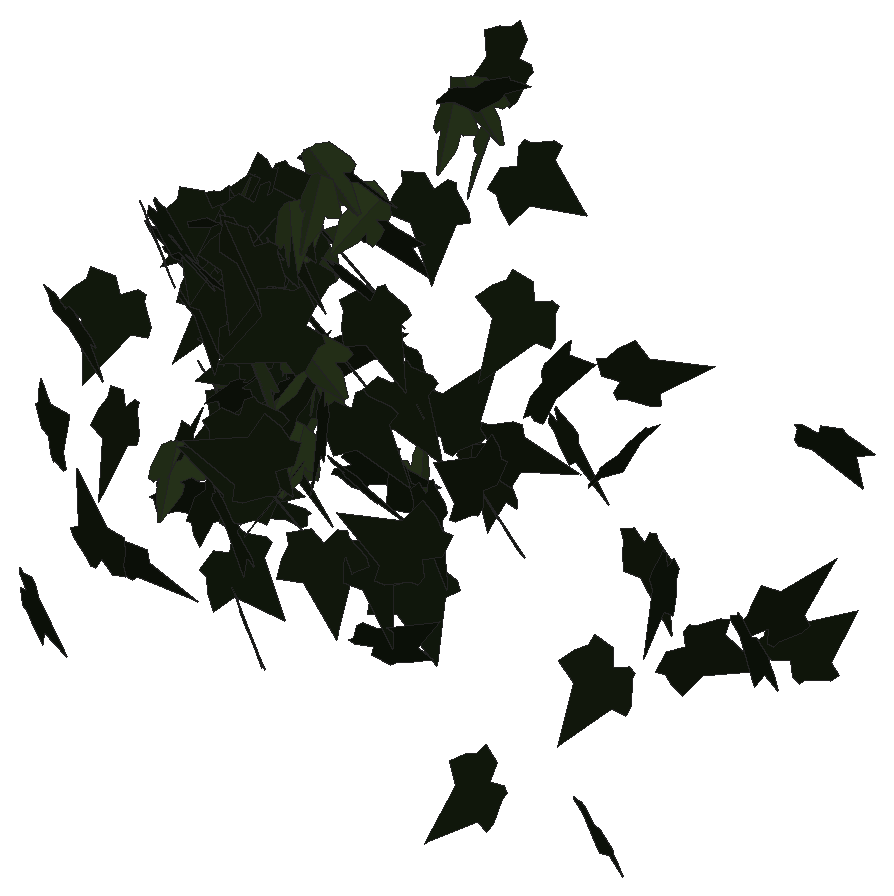
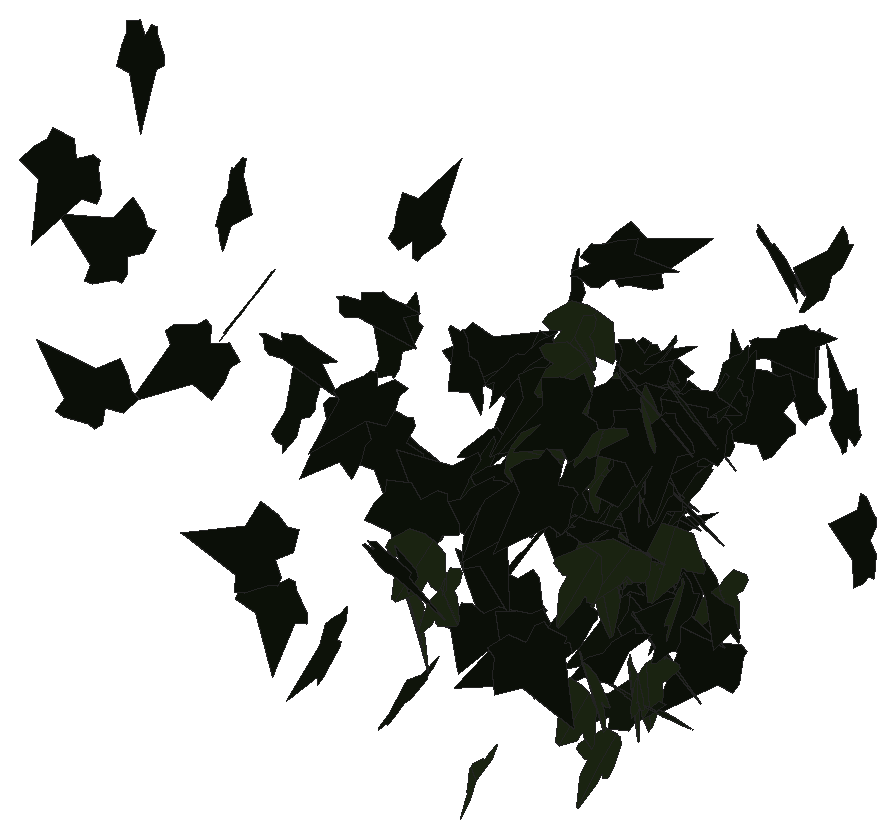
# SketchUp Ruby script. Lengths in inches.
U = 1.inch
M = Sketchup.active_model
def pt(a) = Geom::Point3d.new(a.map { |v| v * U })
def face(e, loops, mat)
  f = e.add_face(loops[0].map { |a| pt(a) })
  loops[1..].each { |l| e.add_face(l.map { |a| pt(a) }).erase! }
  f.material = f.back_material = mat if mat
  f
end
# faces: each face lists its corners as indices into pts; further lists are holes
def faces(e, pts, list, mat = nil) = list.each { |f| face(e, (f[0].is_a?(Array) ? f : [f]).map { |l| l.map { |i| pts[i] } }, mat) }
# xy, xz, yz: faces in a plane at the given z, y or x. An outline is a flat list of corners, or four numbers for a rectangle; further outlines are holes
def ring(l) = l.size == 4 ? [[l[0], l[1]], [l[2], l[1]], [l[2], l[3]], [l[0], l[3]]] : l.each_slice(2).to_a
def flat(e, list, mat, &to3) = list.each { |f| face(e, (f[0].is_a?(Array) ? f : [f]).map { |l| ring(l).map { |u, v| to3.(u, v) } }, mat) }
def xy(e, z, list, mat = nil) = flat(e, list, mat) { |x, y| [x, y, z] }
def xz(e, y, list, mat = nil) = flat(e, list, mat) { |x, z| [x, y, z] }
def yz(e, x, list, mat = nil) = flat(e, list, mat) { |y, z| [x, y, z] }
def lines(e, pts, list) = list.each { |a, b| e.add_line(pt(pts[a]), pt(pts[b])) }
# prism: a flat outline (further loops are holes) pulled along v
def prism(e, loops, v, mat = nil)
  f = face(e, loops, mat); d = Geom::Vector3d.new(v.map { |x| x * U })
  f.pushpull(f.normal.samedirection?(d) ? d.length : -d.length)
end
def box(e, o, s, mat = nil) = prism(e, [[o, [o[0] + s[0], o[1], o[2]], [o[0] + s[0], o[1] + s[1], o[2]], [o[0], o[1] + s[1], o[2]]]], [0, 0, s[2]], mat)
def at(x, y, z, deg = 0) = Geom::Transformation.translation(pt([x, y, z])) * Geom::Transformation.rotation(ORIGIN, Z_AXIS, deg.degrees)
def axes(o, x, y, z) = Geom::Transformation.new([*x, 0, *y, 0, *z, 0, *pt(o).to_a, 1])
def part(name) = M.definitions.add(name)
# library, detail: a bought-in or finely detailed component or shape, given as its bounding box
def library(name, o, s) = part(name).tap { |d| box(d.entities, o, s) }
def detail(e, o, s) = box(e.add_group.entities, o, s)
def put(e, d, t, mat = nil) = e.add_instance(d, t).tap { |i| i.material = mat if mat }
def group(e, t, mat = nil) = e.add_group.tap { |g| g.transformation = t; g.material = mat if mat }.entities
root = M.entities
M.materials.add("efeu1").color = [18, 25, 13]
M.materials.add("efeu2").color = [43, 57, 29]
c1 = part("ivyleaf_10")
p = [[0,0.5,-0.03],[-0.0625,2.02,-0.43],[-0.19,2.01,-0.46],[-0.54,1.05,-0.29],[-0.52,0.625,-0.18],[-0.83,0.76,-0.28],
  [-1.16,0.64,-0.33],[-1.15,0.33,-0.24],[-0.77,-0.39,0.02],[-0.3,-0.51,0.16],[0.04,-0.48,0.23],[-0.02,2.01,-0.4375],
  [-0.06,2.01,-0.43],[0.04,-0.49,0.23],[0.67,-0.49,0.14],[1.38,0.36,-0.2],[1.375,0.51,-0.24],[0.81,0.65,-0.19],
  [0.62,0.59,-0.15],[0.6,1.09,-0.28],[0.5,1.23,-0.31]]
faces(c1.entities,p,[[0,1,2,3,4,5,6,7,8,9,10],[11,12,0,13,14,15,16,17,18,19,20]],"efeu2")
c2 = part("ivyleaf_9")
p = [[1.54,2.16,1.25],[1.36,2.04,1.19],[-0.21,0.99,0.68],[-0.71,1.11,0.82],[-0.85,0.86,0.67],[-0.8,0.17,0.21],
  [-0.9,-0.01,0.1],[-0.67,-0.16,-0.02],[-0.08,-0.08,-0.05],[-0.03,-0.6,-0.4],[0.65,-0.88,-0.66],[0.83,-0.6,-0.49],
  [1.29,-0.42,-0.43],[1.8125,-0.07,-0.26],[1.21,0.44,0.15]]
faces(c2.entities,p,[[0,1,2,3,4,5,6,7,8,9,10,11,12,13,14]],"efeu1")
put(root,c1,axes([53.33,221.73,244.58],[-0.26084,0.4133,0.10556],[-0.07736,0.07585,-0.48812],[-0.4195,-0.27098,0.02438]))
put(root,c1,axes([53.07,223.4,246.125],[0.30993,0.29947,0.2535],[0.18973,0.16837,-0.43087],[-0.34343,0.36327,-0.00928]))
put(root,c1,axes([53.33,223.49,242.65],[-0.0186,0.35996,0.34653],[-0.09177,0.33841,-0.35645],[-0.49115,-0.07687,0.05348]))
put(root,c2,axes([53.1,220.57,248.04],[0.41377,-0.25598,-0.11519],[-0.07624,0.09498,-0.48494],[0.27015,0.41887,0.03957]))
put(root,c1,axes([53.34,221.92,245.64],[-0.47378,-0.13933,-0.07822],[0.06988,0.03944,-0.49352],[0.14369,-0.47857,-0.0179]))
put(root,c2,axes([53.54,220.39,243.92],[-0.03647,0.33293,0.37125],[-0.07657,0.36409,-0.33403],[-0.49276,-0.08121,0.02443]))
put(root,c2,axes([53.12,220.46,247.59],[-0.00979,-0.13779,0.48054],[0.15986,-0.45626,-0.12757],[0.47366,0.15114,0.05298]))
put(root,c2,axes([53.24,221.18,247.5625],[0.42087,0.26197,0.06512],[0.04723,0.04729,-0.49551],[-0.26578,0.42324,0.01506]))
put(root,c1,axes([53.41,223.85,245.99],[0.07815,0.31695,0.37873],[-0.09983,0.38566,-0.30215],[-0.48366,-0.02839,0.12357]))
put(root,c2,axes([53.68,221.22,247.84],[-0.43329,0.24928,0.01071],[-0.00923,0.00543,-0.49989],[-0.24934,-0.43339,-0.0001]))
put(root,c2,axes([53,220.875,247.33],[0.30392,-0.2346,0.32031],[0.28266,-0.15543,-0.38203],[0.27882,0.41329,0.03814]))
put(root,c2,axes([53.57,221.66,246.39],[-0.48347,0.01902,-0.12608],[0.12235,-0.06993,-0.47973],[-0.03588,-0.49472,0.06296]))
put(root,c2,axes([53.52,222.16,247.72],[0.18179,0.42237,-0.19635],[-0.07659,-0.1808,-0.45983],[-0.45944,0.19726,-0.00104]))
put(root,c2,axes([53.08,222.02,244.29],[0.27728,-0.31054,0.27692],[0.18201,-0.20872,-0.41631],[0.37415,0.33166,-0.0027]))
put(root,c1,axes([53.48,227.42,247.08],[0.00599,0.42329,-0.26606],[-0.03576,-0.26503,-0.42247],[-0.49868,0.02409,0.0271]))
put(root,c2,axes([53.61,222.16,246.78],[0.10913,0.48615,-0.04178],[-0.00362,-0.04201,-0.49822],[-0.48793,0.10904,-0.00565]))
put(root,c2,axes([53.49,221.3125,247.93],[-0.34329,-0.32192,-0.16886],[0.14758,0.08884,-0.46939],[0.33222,-0.37212,0.03402]))
put(root,c1,axes([53.48,222.25,243.3],[0.0044,-0.49057,0.09654],[0.15238,-0.09063,-0.46751],[0.47619,0.03353,0.14871]))
put(root,c1,axes([53.54,220.37,243.96],[0.09196,0.44535,-0.20786],[-0.0654,-0.1985,-0.45423],[-0.4871,0.11073,0.02174]))
put(root,c1,axes([53.55,223.64,243.95],[0.40572,-0.2915,-0.02053],[-0.01458,0.0149,-0.49957],[0.29186,0.40596,0.00359]))
put(root,c2,axes([53.42,220.58,243.18],[0.39535,0.29035,0.09693],[0.07144,0.06644,-0.49039],[-0.29765,0.4016,0.01105]))
put(root,c2,axes([53.32,221.4,246.22],[0.12183,-0.41422,0.25214],[0.08363,-0.23814,-0.43162],[0.47767,0.14734,0.01126]))
put(root,c1,axes([53.48,223.98,243.61],[-0.42848,0.15246,-0.20774],[0.17505,-0.12359,-0.45176],[-0.1891,-0.45987,0.05253]))
put(root,c2,axes([53.36,223.12,246.71],[0.06797,-0.42225,0.25901],[0.08983,-0.2466,-0.42558],[0.48715,0.10439,0.04234]))
put(root,c1,axes([53.57,222.15,248.02],[0.24091,-0.40822,0.15913],[0.08605,-0.13398,-0.47397],[0.4296,0.25575,0.0057]))
put(root,c2,axes([53.47,221.53,246.67],[0.01822,-0.4956,-0.06365],[-0.00861,0.06337,-0.49589],[0.49959,0.01916,-0.00623]))
put(root,c2,axes([53.39,217.41,245.63],[-0.05828,0.0526,0.4938],[0.19854,-0.45325,0.07172],[0.45518,0.20444,0.03194]))
put(root,c1,axes([53.67,222.18,246.84],[0.26303,-0.36345,-0.22073],[-0.00674,0.25595,-0.42947],[0.42517,0.2289,0.12975]))
put(root,c2,axes([54.02,221.81,248.09],[-0.3279,0.30737,0.2191],[-0.17435,0.13409,-0.44903],[-0.33479,-0.37087,0.01924]))
put(root,c2,axes([53.97,223.34,246.28],[-0.46479,-0.0286,0.18209],[-0.1759,-0.07874,-0.46137],[0.05506,-0.49293,0.06314]))
put(root,c1,axes([53.7,222.36,243.29],[0.33895,-0.35632,-0.09024],[-0.00109,0.12178,-0.48494],[0.36757,0.32894,0.08177]))
put(root,c2,axes([53.29,222.14,242.67],[0.28974,-0.37151,-0.16743],[0.38414,0.31757,-0.0399],[0.13599,-0.10551,0.46944]))
put(root,c2,axes([53.42,222.03,246.79],[0.47036,-0.16253,0.04837],[0.04593,-0.01519,-0.49765],[0.16324,0.4726,0.00064]))
put(root,c2,axes([54.04,221.54,244.24],[-0.48303,-0.03653,0.12389],[-0.12409,-0.00193,-0.48435],[0.03587,-0.49866,-0.0072]))
put(root,c2,axes([53.64,223.15,244.08],[-0.05725,-0.49668,-0.00567],[-0.00549,0.00634,-0.49993],[0.49668,-0.05718,-0.00618]))
put(root,c2,axes([53.77,218.64,247.67],[-0.30799,-0.39295,-0.02704],[0.01749,0.02065,-0.49927],[0.39349,-0.30849,0.00103]))
put(root,c2,axes([54.13,228.17,247.89],[-0.49045,0.08921,0.03872],[-0.03699,0.01301,-0.49846],[-0.08994,-0.49181,-0.00616]))
put(root,c2,axes([53.62,223.61,245.13],[0.45215,-0.21335,-0.00653],[-0.00106,0.01305,-0.49983],[0.21345,0.45201,0.01134]))
put(root,c2,axes([54.18,224.38,244.56],[-0.00439,0.36922,-0.33713],[-0.11956,-0.32813,-0.35782],[-0.48547,0.07747,0.09117]))
put(root,c2,axes([54.22,221.98,245.89],[-0.43403,0.24559,-0.03615],[0.03102,-0.01859,-0.49869],[-0.24629,-0.43513,0.00091]))
put(root,c1,axes([54.04,227.43,246.61],[0.28328,-0.40788,-0.05818],[-0.03957,0.04335,-0.49654],[0.41011,0.28592,-0.00772]))
put(root,c1,axes([53.91,227.35,247.64],[-0.46349,0.03933,-0.18338],[0.18251,-0.01797,-0.46515],[-0.04318,-0.49813,0.0023]))
put(root,c2,axes([53.63,216.57,243.23],[0.13683,-0.01451,-0.48069],[0.48068,0.01978,0.13623],[0.01507,-0.4994,0.01936]))
put(root,c2,axes([54.33,221.26,243.48],[-0.42259,0.26611,0.02464],[-0.02081,0.0132,-0.49939],[-0.26643,-0.4231,-0.00008]))
put(root,c2,axes([54.27,221.82,246.58],[-0.31397,0.3648,-0.13544],[0.0795,-0.11022,-0.48118],[-0.38092,-0.32369,0.01121]))
put(root,c1,axes([54.14,222.625,245.09],[0.02751,-0.49911,-0.01165],[-0.01666,0.01074,-0.49961],[0.49896,0.02788,-0.01604]))
put(root,c1,axes([53.98,222.84,247.67],[0.28731,0.4007,0.08301],[0.06325,0.05672,-0.49273],[-0.40429,0.29363,-0.0181]))
put(root,c2,axes([53.92,224.05,247.36],[0.49568,0.06435,-0.01283],[-0.01261,-0.00252,-0.49983],[-0.06439,0.49584,-0.00087]))
put(root,c2,axes([54.12,222.37,242.48],[-0.38951,-0.22804,0.21512],[0.1476,-0.43609,-0.19504],[0.27657,-0.08844,0.40704]))
put(root,c2,axes([53.97,222.2,248.21],[-0.04893,-0.29921,-0.39759],[0.08017,0.38955,-0.30302],[0.4911,-0.09341,0.00986]))
put(root,c2,axes([53.94,217.17,248.12],[0.23516,-0.3721,0.23715],[0.15272,-0.18348,-0.43933],[0.41398,0.27906,0.02736]))
put(root,c2,axes([53.94,223.41,246.97],[0.39599,-0.2727,0.13722],[0.12316,-0.06294,-0.48049],[0.27933,0.41434,0.01732]))
put(root,c2,axes([54.43,226.78,248.09],[0.20328,0.44969,-0.08034],[-0.11231,-0.03604,-0.48589],[-0.44279,0.21559,0.08636]))
put(root,c1,axes([54.375,222.43,245.18],[0.10471,0.37847,-0.30951],[-0.10735,-0.29101,-0.39216],[-0.47698,0.14858,0.02031]))
put(root,c2,axes([54.18,221.6,248.17],[0.10974,-0.40117,-0.27753],[-0.00425,0.28366,-0.41172],[0.48779,0.09273,0.05885]))
put(root,c2,axes([54.11,223.22,248.24],[0.47991,-0.01243,0.13974],[0.14028,0.03661,-0.47852],[0.00166,0.4985,0.03863]))
put(root,c2,axes([54.48,220.01,243.85],[0.0486,-0.05914,-0.49411],[-0.31187,0.38325,-0.07654],[0.38778,0.31564,0.00036]))
put(root,c2,axes([54.84,221.01,246.22],[-0.35937,0.20451,0.28112],[-0.25071,0.12762,-0.41335],[-0.24082,-0.43805,0.01082]))
put(root,c2,axes([54.66,220.83,245.53],[-0.02191,0.46774,-0.17533],[-0.06885,-0.17665,-0.46266],[-0.49475,0.00387,0.07215]))
put(root,c2,axes([54.7,220.8,247.98],[-0.1845,0.46439,0.01744],[-0.02466,0.00895,-0.49931],[-0.46406,-0.18511,0.0196]))
put(root,c2,axes([54.2,222.14,247.45],[0.34163,-0.36318,0.03734],[0.04068,-0.01296,-0.49817],[0.36282,0.34342,0.02069]))
put(root,c2,axes([54.9,221.09,245.91],[-0.4459,0.10083,0.2025],[-0.19608,0.05095,-0.45712],[-0.11282,-0.48707,-0.0059]))
put(root,c1,axes([54.56,222.03,247.89],[-0.01053,0.48786,-0.10899],[0.00877,-0.10882,-0.48794],[-0.49981,-0.01218,-0.00626]))
put(root,c2,axes([54.4,221.03,247.93],[0.18131,-0.45741,0.0889],[0.04038,-0.0796,-0.49197],[0.46422,0.18558,0.00808]))
put(root,c2,axes([54.39,221.96,243.74],[0.40252,-0.29647,0.0091],[0.00725,-0.0055,-0.49992],[0.29652,0.40258,-0.00013]))
put(root,c2,axes([54.5,221.03,243.86],[0.4652,-0.18302,-0.00974],[-0.00895,0.00386,-0.49991],[0.18306,0.46528,0.00031]))
put(root,c2,axes([54.68,220.87,247.875],[-0.15741,-0.47089,0.059],[0.02925,-0.07167,-0.49397],[0.47367,-0.15207,0.05011]))
put(root,c1,axes([54.61,222.7,248.66],[-0.36688,0.06225,-0.33395],[0.32165,-0.09445,-0.37098],[-0.10927,-0.48704,0.02926]))
put(root,c1,axes([54.86,223.67,247.49],[-0.14331,-0.2021,0.4343],[0.04712,-0.45707,-0.19715],[0.4767,-0.01558,0.15005]))
put(root,c2,axes([55.03,221.67,245.6875],[-0.16166,0.45962,-0.11232],[0.02473,-0.11032,-0.48705],[-0.4725,-0.16303,0.01294]))
put(root,c2,axes([54.73,223.89,246.9375],[0.48128,0.13322,-0.02501],[-0.02795,0.00728,-0.49916],[-0.13264,0.48187,0.01446]))
put(root,c1,axes([55.03,224.58,241.98],[0.00583,0.33314,-0.37281],[-0.095,0.36678,0.32626],[0.49086,0.06703,0.06757]))
put(root,c1,axes([54.85,221.8,246.26],[0.01127,-0.25592,0.42939],[0.26963,-0.35855,-0.22078],[0.42092,0.23653,0.12992]))
put(root,c2,axes([55.42,220.23,244.21],[-0.22494,-0.37723,-0.23895],[-0.12159,-0.2057,0.43921],[-0.42967,0.2557,0.0008]))
put(root,c2,axes([54.99,225.02,247.18],[-0.04637,-0.49664,-0.03469],[0.00848,0.03405,-0.49877],[0.49777,-0.04685,0.00527]))
put(root,c1,axes([55.15,221.96,248.61],[-0.00504,0.40423,-0.29423],[-0.03699,-0.29374,-0.40293],[-0.4986,0.01771,0.03286]))
put(root,c1,axes([55.22,221.32,244.46],[0.48837,-0.10362,-0.02762],[-0.02804,0.00094,-0.49921],[0.10351,0.48914,-0.00489]))
put(root,c2,axes([55.56,215.99,244.85],[0.29204,-0.15673,0.37437],[-0.23434,0.31144,0.31319],[-0.33136,-0.35838,0.10845]))
put(root,c1,axes([55.41,220.07,246.42],[-0.39675,0.27675,-0.12648],[0.10901,-0.06476,-0.48365],[-0.28408,-0.41136,-0.00895]))
put(root,c2,axes([55.27,222.72,243.4],[0.39786,0.16645,0.25299],[0.23414,0.09585,-0.43127],[-0.19207,0.46164,-0.00167]))
put(root,c2,axes([55.79,219.96,244.12],[-0.0776,0.45882,0.18294],[-0.02834,0.18074,-0.46533],[-0.49313,-0.08259,-0.00204]))
put(root,c2,axes([55.32,219.57,243.79],[0.11605,-0.31862,0.36745],[0.12893,-0.34409,-0.33908],[0.46894,0.17345,0.0023]))
put(root,c2,axes([55.48,219.37,243.32],[0.12182,-0.28213,-0.39441],[-0.08833,0.38695,-0.30408],[0.47682,0.14376,0.04444]))
put(root,c2,axes([56.08,220.21,245.68],[-0.24216,0.39801,0.18151],[-0.08724,0.15936,-0.46583],[-0.42866,-0.25728,-0.00774]))
put(root,c2,axes([55.67,221.85,247.42],[0.49702,-0.0426,-0.03395],[-0.02983,0.04795,-0.4968],[0.04558,0.49587,0.04513]))
put(root,c2,axes([55.88,216.14,247.48],[-0.38974,-0.01168,-0.31299],[0.31319,-0.02046,-0.38922],[-0.00372,-0.49944,0.02327]))
put(root,c2,axes([55.59,216.36,244.73],[0.44488,-0.0543,0.22166],[0.2192,-0.03347,-0.44814],[0.0635,0.49591,-0.00597]))
put(root,c2,axes([56.29,218.59,246.4],[-0.11587,-0.17492,-0.45385],[0.26795,0.36641,-0.20963],[0.40593,-0.29179,0.00883]))
put(root,c2,axes([56.41,224.6875,242.92],[0.0248,-0.41546,0.27709],[0.08596,-0.26974,-0.41213],[0.49193,0.06808,0.05804]))
put(root,c2,axes([57.06,219.14,248.1],[-0.33774,-0.21632,0.29856],[-0.25124,-0.16129,-0.40108],[0.26983,-0.42094,0.00025]))
put(root,c1,axes([56.81,219.65,247.34],[-0.42311,-0.1301,-0.2325],[0.22112,0.07193,-0.44264],[0.14862,-0.47739,-0.00333]))
put(root,c2,axes([56.82,222.15,245.96],[0.37233,-0.1689,-0.28783],[-0.23254,0.178,-0.40526],[0.23937,0.43565,0.054]))
put(root,c2,axes([56.79,221.23,247.46],[0.13211,-0.44477,-0.18634],[-0.01814,0.18849,-0.46276],[0.48189,0.12903,0.03367]))
put(root,c2,axes([57.04,217.67,243.57],[0.34526,-0.07677,-0.35341],[-0.34467,0.07813,-0.35369],[0.10953,0.48785,0.00103]))
put(root,c2,axes([56.91,224.81,248.4],[0.1064,-0.16964,-0.45815],[-0.06396,0.46002,-0.18518],[0.48434,0.09802,0.07619]))
put(root,c2,axes([57.34,221.5,244.34],[0.16069,0.12281,-0.45727],[-0.45143,-0.10589,-0.18708],[-0.14279,0.47298,0.07685]))
put(root,c2,axes([56.98,219.8,243.82],[-0.23913,-0.31437,-0.30657],[0.21538,0.22023,-0.39384],[0.38265,-0.32042,0.03009]))
put(root,c2,axes([57.09,221.45,246.01],[0.11132,-0.36514,-0.32293],[-0.02743,0.32603,-0.37809],[0.48668,0.10189,0.05256]))
put(root,c2,axes([57.18,220.3,246.09],[-0.11634,-0.09643,-0.47662],[0.32866,0.3456,-0.15014],[0.35839,-0.34823,-0.01703]))
put(root,c2,axes([57.4,221.49,242.7],[-0.17278,-0.33227,-0.33128],[0.15296,0.29385,-0.37451],[0.44357,-0.23076,0.00011]))
put(root,c2,axes([57.37,220.47,243.46],[0.1721,-0.46935,-0.00973],[-0.00828,0.00733,-0.49988],[0.46937,0.17222,-0.00525]))
put(root,c2,axes([57.49,222.12,245.05],[-0.17805,-0.05549,0.46392],[0.43319,0.16642,0.18616],[-0.17507,0.46822,-0.01119]))
put(root,c2,axes([57.47,225.12,243.82],[0.39943,-0.27719,-0.11673],[-0.09639,0.06584,-0.48618],[0.2849,0.41089,-0.00084]))
put(root,c2,axes([58.1,217.07,246.8],[-0.11473,-0.02036,0.48623],[-0.47803,-0.08892,-0.11652],[0.09122,-0.49161,0.00094]))
put(root,c2,axes([57.65,220.29,242.07],[0.39905,0.26857,-0.13651],[0.11369,0.07556,0.481],[0.27899,-0.41493,-0.00076]))
put(root,c2,axes([57.93,218.59,247.08],[-0.03632,-0.03455,-0.49748],[0.44713,-0.22312,-0.01715],[-0.22081,-0.44612,0.0471]))
put(root,c2,axes([57.98,219.1875,245.7],[0.35799,-0.24908,0.24454],[0.23895,-0.08048,-0.43177],[0.25446,0.426,0.06141]))
put(root,c2,axes([58.99,224.68,244.04],[-0.02152,0.49287,0.08133],[-0.00346,0.08126,-0.49334],[-0.49952,-0.02179,-0.00009]))
put(root,c2,axes([59.02,222.78,246.18],[-0.04838,0.15201,-0.47387],[-0.26495,0.39515,0.1538],[0.42126,0.26599,0.04231]))
put(root,c2,axes([58.61,225.28,244.98],[0.17368,0.00786,0.4688],[0.46695,0.04231,-0.1737],[-0.0424,0.49814,0.00736]))
put(root,c2,axes([59.26,222.13,247.95],[-0.44196,-0.23156,-0.03242],[0.03346,0.00598,-0.49884],[0.23142,-0.44311,0.01021]))
put(root,c2,axes([58.79,221.77,245.4375],[0.126,0.12747,-0.46677],[0.30777,0.35108,0.17895],[0.37337,-0.33241,0.01001]))
put(root,c2,axes([59.77,218.67,245.12],[-0.05572,0.0422,0.49509],[-0.49292,-0.0675,-0.04972],[0.06264,-0.49362,0.04913]))
put(root,c2,axes([59.38,219.38,245.71],[-0.16842,-0.00292,-0.47077],[0.46823,0.05091,-0.16782],[0.04891,-0.49739,-0.01441]))
put(root,c2,axes([60.43,219.76,245.66],[0.14403,-0.27295,0.39339],[0.22319,-0.32517,-0.30733],[0.42361,0.26413,0.02817]))
put(root,c2,axes([61.14,218.54,246.88],[0.06426,0.0663,0.4914],[-0.2977,-0.39111,0.0917],[0.39654,-0.30436,-0.01079]))
put(root,c2,axes([62.07,217.52,242.36],[-0.49901,0.03067,-0.00677],[0.00676,-0.00041,-0.49995],[-0.03068,-0.49906,0]))
put(root,c2,axes([63.08,220.22,245.78],[0.21159,-0.45287,0.01194],[0.00087,-0.01277,-0.49984],[0.45302,0.21154,-0.00462]))
put(root,c2,axes([63.46,218.85,244.3],[-0.47278,-0.15055,-0.06174],[0.05946,0.01673,-0.49617],[0.15146,-0.4765,0.00208]))
put(root,c2,axes([64.17,219.9375,244.48],[0.00844,0.02623,-0.49924],[-0.01574,0.49908,0.02596],[0.49968,0.01528,0.00925]))
put(root,c2,axes([64.1,217.67,242.25],[0.35792,-0.14114,-0.31934],[0.29392,-0.12502,0.38468],[-0.18844,-0.46309,-0.00653]))
put(root,c2,axes([64.65,218.77,246.51],[-0.056,0.05708,-0.49356],[0.39446,-0.29689,-0.07909],[-0.3021,-0.39824,-0.01178]))
put(root,c2,axes([64.96,221.5625,243.86],[-0.11021,-0.0001,0.4877],[0.47812,-0.09867,0.10802],[0.09622,0.49017,0.02184]))
put(root,c2,axes([65.51,221.58,248.04],[0.44331,0.20439,-0.10817],[-0.09648,-0.04909,-0.48814],[-0.21016,0.45367,-0.00408]))
put(root,c2,axes([65.87,219.87,245.5],[0.00817,-0.0931,0.49119],[0.40904,0.28369,0.04697],[-0.28743,0.40106,0.0808]))
put(root,c2,axes([67.89,216.85,247.3],[0.3086,0.02973,-0.39228],[-0.39146,-0.02623,-0.30995],[-0.03901,0.49843,0.00709]))
